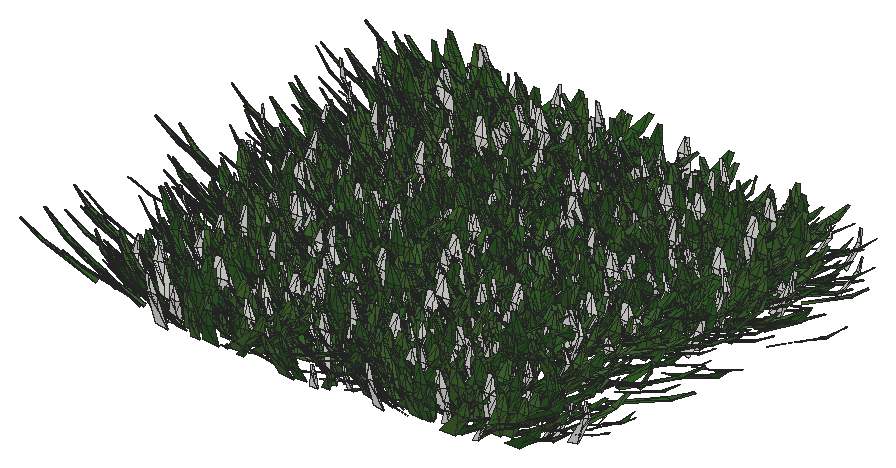
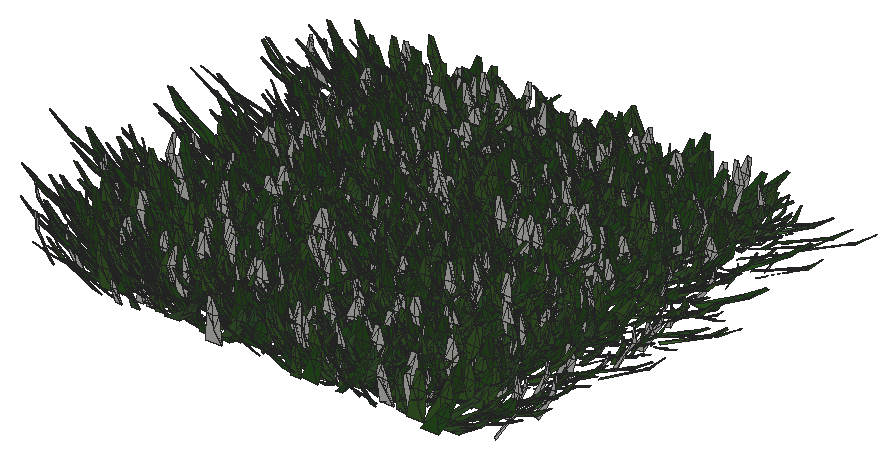
# SketchUp Ruby script. Lengths in inches.
U = 1.inch
M = Sketchup.active_model
def pt(a) = Geom::Point3d.new(a.map { |v| v * U })
def face(e, loops, mat)
  f = e.add_face(loops[0].map { |a| pt(a) })
  loops[1..].each { |l| e.add_face(l.map { |a| pt(a) }).erase! }
  f.material = f.back_material = mat if mat
  f
end
# faces: each face lists its corners as indices into pts; further lists are holes
def faces(e, pts, list, mat = nil) = list.each { |f| face(e, (f[0].is_a?(Array) ? f : [f]).map { |l| l.map { |i| pts[i] } }, mat) }
# xy, xz, yz: faces in a plane at the given z, y or x. An outline is a flat list of corners, or four numbers for a rectangle; further outlines are holes
def ring(l) = l.size == 4 ? [[l[0], l[1]], [l[2], l[1]], [l[2], l[3]], [l[0], l[3]]] : l.each_slice(2).to_a
def flat(e, list, mat, &to3) = list.each { |f| face(e, (f[0].is_a?(Array) ? f : [f]).map { |l| ring(l).map { |u, v| to3.(u, v) } }, mat) }
def xy(e, z, list, mat = nil) = flat(e, list, mat) { |x, y| [x, y, z] }
def xz(e, y, list, mat = nil) = flat(e, list, mat) { |x, z| [x, y, z] }
def yz(e, x, list, mat = nil) = flat(e, list, mat) { |y, z| [x, y, z] }
def lines(e, pts, list) = list.each { |a, b| e.add_line(pt(pts[a]), pt(pts[b])) }
# prism: a flat outline (further loops are holes) pulled along v
def prism(e, loops, v, mat = nil)
  f = face(e, loops, mat); d = Geom::Vector3d.new(v.map { |x| x * U })
  f.pushpull(f.normal.samedirection?(d) ? d.length : -d.length)
end
def box(e, o, s, mat = nil) = prism(e, [[o, [o[0] + s[0], o[1], o[2]], [o[0] + s[0], o[1] + s[1], o[2]], [o[0], o[1] + s[1], o[2]]]], [0, 0, s[2]], mat)
def at(x, y, z, deg = 0) = Geom::Transformation.translation(pt([x, y, z])) * Geom::Transformation.rotation(ORIGIN, Z_AXIS, deg.degrees)
def axes(o, x, y, z) = Geom::Transformation.new([*x, 0, *y, 0, *z, 0, *pt(o).to_a, 1])
def part(name) = M.definitions.add(name)
# library, detail: a bought-in or finely detailed component or shape, given as its bounding box
def library(name, o, s) = part(name).tap { |d| box(d.entities, o, s) }
def detail(e, o, s) = box(e.add_group.entities, o, s)
def put(e, d, t, mat = nil) = e.add_instance(d, t).tap { |i| i.material = mat if mat }
def group(e, t, mat = nil) = e.add_group.tap { |g| g.transformation = t; g.material = mat if mat }.entities
root = M.entities
M.materials.add("Material10").color = [48, 100, 38]
M.materials.add("Material3").color = [68, 110, 58]
M.materials.add("Material4").color = [48, 90, 38]
M.materials.add("Material5").color = [68, 110, 48]
M.materials.add("Material6").color = [48, 90, 48]
M.materials.add("Material7").color = [58, 110, 58]
M.materials.add("Material8").color = [58, 90, 38]
M.materials.add("Material9").color = [68, 100, 58]
c1 = part("grass00")
p = [[-0.6875,0.15,0],[-0.56,0.08,5.52],[-0.04,0.03,2.76],[0.48,-0.02,0],[0.35,-0.02,5.52],[-0.1,-0.14,5.52],
  [-0.12,0.65,8.37],[-0.42,0.65,8.37]]
faces(c1.entities,p,[[0,1,2,3],[3,2,4],[1,5,2],[5,4,2],[1,6,5],[4,5,6],[7,6,1]])
c2 = part("Group16\#1")
put(c2.entities,c1,axes([1.44,-0.61,-0.01],[0.05352,0.12609,0],[-0.10704,0.04543,0.07239],[0.06664,-0.02828,0.11628]),"Material6")
put(c2.entities,c1,axes([0.76,-0.15,-0.01],[0.04676,0.24062,0],[-0.23162,0.04501,0.06642],[0.0652,-0.01267,0.23595]),"Material3")
put(c2.entities,c1,axes([0.79,0.01,-0.01],[-0.00606,0.34651,0],[-0.34381,-0.00602,0.0432],[0.04319,0.00076,0.34386]))
put(c2.entities,c1,axes([1,0.23,-0.01],[-0.07192,0.31144,0],[-0.28722,-0.06632,0.1236],[0.12043,0.02781,0.29478]),"Material5")
put(c2.entities,c1,axes([1.66,0.77,-0.01],[-0.13828,0.29651,0],[-0.21551,-0.1005,0.22471],[0.20365,0.09498,0.23779]),"Material10")
put(c2.entities,c1,axes([0.6875,0.52,-0.01],[-0.18126,0.24051,0],[-0.22746,-0.17142,0.09788],[0.07817,0.05891,0.28481]),"Material5")
put(c2.entities,c1,axes([0.68,0.78,-0.01],[-0.215,0.18688,0],[-0.12385,-0.14248,0.21334],[0.13995,0.16101,0.18878]),"Material3")
put(c2.entities,c1,axes([0.56,1,-0.01],[-0.13756,0.07624,0],[-0.06159,-0.11112,0.0927],[0.04494,0.08108,0.12705]),"Material5")
put(c2.entities,c1,axes([0.2,0.64,-0.01],[-0.23729,0.07254,0],[-0.05711,-0.18681,0.153],[0.04473,0.14632,0.19535]),"Material10")
put(c2.entities,c1,axes([0.0625,0.72,-0.01],[-0.28874,0.02525,0],[-0.02179,-0.24916,0.14647],[0.01276,0.14591,0.25012]),"Material3")
put(c2.entities,c1,axes([-0.08,0.62,-0.01],[-0.34089,-0.04187,0],[0.03255,-0.26504,0.216],[-0.02633,0.21439,0.26703]),"Material10")
put(c2.entities,c1,axes([-0.34,0.98,-0.01],[-0.14314,-0.0493,0],[0.04397,-0.12769,0.06843],[-0.02228,0.0647,0.13505]),"Material10")
put(c2.entities,c1,axes([-0.87,1.45,-0.01],[-0.23488,-0.14114,0],[0.13761,-0.22901,0.06087],[-0.03135,0.05217,0.26717]))
put(c2.entities,c1,axes([-0.72,0.77,-0.01],[-0.14208,-0.13251,0],[0.07209,-0.0773,0.16301],[-0.11118,0.11922,0.1057]),"Material10")
put(c2.entities,c1,axes([-0.62,0.43,-0.01],[-0.14845,-0.21203,0],[0.18654,-0.13061,0.12304],[-0.10079,0.07057,0.22772]),"Material3")
put(c2.entities,c1,axes([-0.68,0.29,-0.01],[-0.13639,-0.32136,0],[0.31723,-0.13464,0.05579],[-0.05136,0.0218,0.34462]),"Material4")
put(c2.entities,c1,axes([-0.64,0.125,-0.01],[-0.0458,-0.23569,0],[0.22124,-0.043,0.08276],[-0.08124,0.01579,0.22538]),"Material7")
put(c2.entities,c1,axes([-1.6,-0.03,-0.01],[0.00576,-0.32897,0],[0.27526,0.00482,0.18018],[-0.18015,-0.00315,0.2753]),"Material5")
put(c2.entities,c1,axes([-1.36,-0.31,-0.01],[0.05718,-0.24765,0],[0.18172,0.04196,0.17267],[-0.16825,-0.03885,0.1865]),"Material10")
put(c2.entities,c1,axes([-1.54,-0.72,-0.01],[0.06537,-0.14017,0],[0.13555,0.06321,0.03939],[-0.0357,-0.01665,0.14956]))
put(c2.entities,c1,axes([-1.19,-0.9,-0.01],[0.09597,-0.12735,0],[0.11214,0.08451,0.07557],[-0.06035,-0.04548,0.14042]),"Material9")
put(c2.entities,c1,axes([-0.47,-0.54,-0.01],[0.11588,-0.10072,0],[0.0618,0.0711,0.12124],[-0.07953,-0.0915,0.0942]))
put(c2.entities,c1,axes([-0.47,-0.84,-0.01],[0.11927,-0.0661,0],[0.06603,0.11913,0.00646],[-0.00313,-0.00565,0.13621]),"Material5")
put(c2.entities,c1,axes([-0.38,-1.24,-0.01],[0.28037,-0.08571,0],[0.0618,0.20215,0.20315],[-0.05939,-0.19428,0.21139]),"Material9")
put(c2.entities,c1,axes([-0.06,-0.66,-0.01],[0.22719,-0.01987,0],[0.01247,0.14255,0.17758],[-0.01547,-0.17691,0.1431]),"Material8")
put(c2.entities,c1,axes([0.11,-0.89,-0.01],[0.14882,0.01828,0],[-0.01058,0.08611,0.12229],[0.01491,-0.12138,0.08676]),"Material6")
put(c2.entities,c1,axes([0.25,-0.72,-0.01],[0.20481,0.07053,0],[-0.06206,0.18022,0.10291],[0.03351,-0.0973,0.1906]),"Material6")
put(c2.entities,c1,axes([0.85,-1.42,-0.01],[0.16481,0.09904,0],[-0.09472,0.15762,0.05616],[0.02893,-0.04814,0.18389]),"Material5")
put(c2.entities,c1,axes([1.01,-1.09,-0.01],[0.21858,0.20385,0],[-0.17495,0.1876,0.15339],[0.10462,-0.11218,0.25652]),"Material10")
put(c2.entities,c1,axes([1.01,-0.71,-0.01],[0.08733,0.12473,0],[-0.06445,0.04512,0.13037],[0.1068,-0.07477,0.07867]),"Material6")
c3 = part("Group15\#1")
put(c3.entities,c2,at(0,0,0))
c4 = part("3darcstudiotree_grass00\#1")
put(c4.entities,c3,at(0,0,0))
put(root,c4,axes([193.53,26.9,7.6],[-2.68493,-0.72179,0],[2.74212,-0.63751,-0.03633],[0.19715,-0.04583,1.73438]))
put(root,c4,axes([193.63,25.22,7.6],[-1.94469,-0.81082,0],[3.41072,-0.51128,-0.04451],[0.23926,-0.03587,1.55797]))
put(root,c4,axes([194.18,17.8125,7.6],[-4.38536,-0.48819,0],[1.68539,-0.94622,-0.04343],[0.09225,-0.05179,1.35201]))
put(root,c4,axes([193.89,13.31,7.6],[-0.93763,-1.01509,0],[3.58265,-0.20683,-0.0292],[0.19066,-0.01101,1.53984]))
put(root,c4,axes([193.6,18.74,7.6],[2.32628,-1.10135,0],[3.26689,0.43127,-0.03491],[0.22091,0.02916,1.65255]))
put(root,c4,axes([194.4,5.27,7.6],[-3.78007,0.18751,0],[-0.9942,-1.25267,-0.05548],[-0.05563,-0.0701,1.6451]))
put(root,c4,axes([195.64,33.04,7.6],[-3.41877,-0.81095,0],[3.11222,-0.82002,-0.00166],[0.00704,-0.00186,1.74215]))
put(root,c4,axes([193.625,37.75,7.6],[3.56011,0.3766,0],[-1.5529,0.91751,-0.02719],[-0.08207,0.04849,1.929]))
put(root,c4,axes([193.64,38.23,7.6],[-0.28146,1.0454,0],[-4.85505,-0.0817,-0.01753],[-0.10805,-0.00182,1.87889]))
put(root,c4,axes([193.54,23.21,7.6],[4.34869,0.47354,0],[-1.70545,0.97885,-0.04191],[-0.08317,0.04774,1.32656]))
put(root,c4,axes([194.17,42.1875,7.6],[0.50605,0.98572,0],[-4.41784,0.14175,-0.0516],[-0.36721,0.01178,1.99718]))
put(root,c4,axes([193.98,29.9,7.6],[4.51798,0.20316,0],[-0.79252,1.10155,-0.03729],[-0.03789,0.05267,1.60628]))
put(root,c4,axes([195.89,11.21,7.6],[-4.34417,-0.18262,0],[0.70687,-1.05094,-0.0114],[0.01401,-0.02082,1.97478]))
put(root,c4,axes([194.25,27.89,7.6],[2.21014,1.15532,0],[-3.78234,0.45223,-0.02212],[-0.14871,0.01778,1.95299]))
put(root,c4,axes([194.5625,16.51,7.6],[-0.29005,1.03921,0],[-4.26068,-0.07432,-0.02357],[-0.13601,-0.00237,1.54387]))
put(root,c4,axes([194.57,9.76,7.6],[4.64548,-0.02052,0],[0.0884,1.25077,-0.02875],[0.00253,0.03584,1.55972]))
put(root,c4,axes([194.73,34.38,7.6],[2.69774,0.60172,0],[-2.53829,0.71125,-0.00625],[-0.03018,0.00846,1.72796]))
put(root,c4,axes([196.32,21.58,7.6],[-4.15604,0.63305,0],[-2.33124,-0.95655,-0.05764],[-0.19304,-0.07921,1.8024]))
put(root,c4,axes([196.75,6.94,7.6],[1.24811,-0.98204,0],[4.93225,0.39179,-0.03698],[0.19941,0.01584,1.82987]))
put(root,c4,axes([197.36,14.11,7.6],[-2.73285,-0.87798,0],[3.13409,-0.60971,-0.01663],[0.09994,-0.01944,1.89037]))
put(root,c4,axes([196.96,4.1,7.6],[-3.26487,0.7652,0],[-2.88539,-0.76944,-0.04557],[-0.23173,-0.0618,1.96028]))
put(root,c4,axes([196.54,30.82,7.6],[-2.34155,0.84913,0],[-3.4682,-0.59774,-0.02321],[-0.12342,-0.02127,1.70026]))
put(root,c4,axes([197.26,8.99,7.6],[-3.68799,0.26675,0],[-1.34322,-1.16069,-0.00573],[-0.00843,-0.00729,1.59925]))
put(root,c4,axes([197.2,36.07,7.6],[2.33049,-0.73294,0],[3.96124,0.7872,-0.06111],[0.26943,0.05354,1.78135]))
put(root,c4,axes([197.32,40.72,7.6],[3.80611,-0.44418,0],[1.98468,1.06289,-0.02938],[0.0699,0.03743,1.64954]))
put(root,c4,axes([197.125,20.72,7.6],[5.11514,-0.08131,0],[0.26106,1.02638,-0.03177],[0.01497,0.05885,1.90853]))
put(root,c4,axes([199.55,25.45,7.6],[-4.00581,-0.59681,0],[2.18474,-0.9165,-0.01663],[0.06212,-0.02606,1.94585]))
put(root,c4,axes([199.72,4.14,7.6],[3.537,-0.94689,0],[2.76209,0.64485,-0.01281],[0.06208,0.01449,1.56626]))
put(root,c4,axes([201.32,22.05,7.6],[-1.77,-0.83286,0],[4.02387,-0.53447,-0.00698],[0.04087,-0.00543,1.8873]))
put(root,c4,axes([200.93,6.76,7.6],[1.67638,-1.0425,0],[4.59893,0.4622,-0.01772],[0.09487,0.00953,1.7874]))
put(root,c4,axes([201.5,13.21,7.6],[-3.4263,-0.91381,0],[3.1573,-0.73989,-0.03051],[0.13581,-0.03183,1.65027]))
put(root,c4,axes([200.84,39.84,7.6],[2.30637,-1.06411,0],[3.89478,0.5276,-0.00988],[0.05923,0.00802,1.88737]))
put(root,c4,axes([199.71,17.35,7.6],[5.17876,0.00972,0],[-0.03633,1.20929,-0.012],[-0.00051,0.01694,1.70791]))
put(root,c4,axes([200.52,5.41,7.6],[3.44483,-0.53348,0],[2.02838,0.81862,-0.00486],[0.01517,0.00612,1.42853]))
put(root,c4,axes([199.85,19.01,7.6],[1.61317,1.05687,0],[-3.89248,0.37133,-0.03212],[-0.19954,0.01904,1.73128]))
put(root,c4,axes([200.26,9.9,7.6],[4.23132,0.05428,0],[-0.26252,1.27912,-0.05168],[-0.01396,0.06804,1.68853]))
put(root,c4,axes([200.07,14.6,7.6],[0.18775,1.28338,0],[-5.04354,0.04611,-0.0182],[-0.08343,0.00076,1.44668]))
put(root,c4,axes([200.24,27.72,7.6],[0.66659,0.99759,0],[-3.70369,0.15468,-0.00028],[-0.00179,0.00007,1.50491]))
put(root,c4,axes([200.59,38.79,7.6],[-0.12653,1.00906,0],[-4.40907,-0.03456,-0.04067],[-0.22619,-0.00177,1.53414]))
put(root,c4,axes([201.48,32.94,7.6],[-3.44749,0.85218,0],[-2.82175,-0.71346,-0.03762],[-0.15511,-0.03922,1.47105]))
put(root,c4,axes([200.23,36.24,7.6],[0.53467,1.10303,0],[-5.00046,0.15149,-0.01569],[-0.0735,0.00223,1.48562]))
put(root,c4,axes([202.59,29.92,7.6],[-3.66347,-0.90665,0],[3.59625,-0.9082,-0.03717],[0.1584,-0.04,1.93537]))
put(root,c4,axes([202.37,26.35,7.6],[-4.4143,-0.18542,0],[0.67487,-1.00419,-0.01654],[0.02043,-0.03039,1.89711]))
put(root,c4,axes([202.8,30.91,7.6],[-1.79213,-0.89815,0],[3.71156,-0.46287,-0.00448],[0.02956,-0.00369,1.90991]))
put(root,c4,axes([201.9,16.58,7.6],[-3.49749,0.50247,0],[-2.5408,-1.10534,-0.04948],[-0.12396,-0.05393,1.60238]))
put(root,c4,axes([201.3,34.43,7.6],[0.73607,0.9032,0],[-4.03456,0.2055,-0.04728],[-0.29589,0.01507,1.64346]))
put(root,c4,axes([201.66,23.49,7.6],[3.54729,0.43846,0],[-1.7678,0.89387,-0.03066],[-0.09543,0.04825,1.75054]))
put(root,c4,axes([202.87,8.96,7.6],[0.42302,-0.9917,0],[3.83549,0.10225,-0.04937],[0.35058,0.00935,1.72169]))
put(root,c4,axes([203.12,20.35,7.6],[-1.77196,1.05602,0],[-3.98674,-0.4181,-0.04701],[-0.29505,-0.03094,1.83905]))
put(root,c4,axes([203.33,11.55,7.6],[0.45093,1.12107,0],[-3.84241,0.0966,-0.04963],[-0.30261,0.00761,1.47912]))
put(root,c4,axes([202.64,41.44,7.6],[3.32772,0.78374,0],[-3.41591,0.90649,-0.01047],[-0.04436,0.01177,1.92288]))
put(root,c4,axes([203.77,36.9,7.6],[4.23567,0.36269,0],[-1.24548,0.90909,-0.02009],[-0.04731,0.03453,1.7458]))
put(root,c4,axes([205.65,36.125,7.6],[-4.4227,-0.30365,0],[1.03811,-0.94502,-0.02848],[0.05651,-0.05144,1.83531]))
put(root,c4,axes([205.36,40.33,7.6],[-0.43672,-1.24202,0],[4.36716,-0.09597,-0.04765],[0.30496,-0.0067,1.76037]))
put(root,c4,axes([205.6,42.0625,7.6],[-4.11211,0.64037,0],[-1.92557,-0.77282,-0.01072],[-0.04599,-0.01846,1.84718]))
put(root,c4,axes([206.2,14.46,7.6],[-4.34593,0.58001,0],[-2.21528,-1.03742,-0.03463],[-0.1032,-0.04833,1.86049]))
put(root,c4,axes([205.74,19.26,7.6],[-1.86227,1.06204,0],[-3.42788,-0.37567,-0.01229],[-0.09526,-0.01044,1.9803]))
put(root,c4,axes([207.29,34.14,7.6],[-3.5926,-0.75101,0],[3.19063,-0.95393,-0.04137],[0.11689,-0.03495,1.36909]))
put(root,c4,axes([206.76,28.27,7.6],[3.48166,-0.50059,0],[2.44605,1.06327,-0.03788],[0.08627,0.0375,1.40078]))
put(root,c4,axes([206.13,26.41,7.6],[4.43547,0.23328,0],[-0.86743,1.0308,-0.04482],[-0.053,0.06298,1.51278]))
put(root,c4,axes([208.07,37.01,7.6],[-3.11664,-0.68281,0],[2.49826,-0.71269,-0.01406],[0.06937,-0.01979,1.77353]))
put(root,c4,axes([207.15,32.86,7.6],[4.18182,-0.37358,0],[1.54336,1.07977,-0.0155],[0.03636,0.02544,1.9985]))
put(root,c4,axes([208.6,10.53,7.6],[-2.65841,-0.80925,0],[2.97739,-0.6113,-0.021],[0.09455,-0.01941,1.40308]))
put(root,c4,axes([208.53,15.63,7.6],[-1.89766,-0.97867,0],[3.50817,-0.42515,-0.03263],[0.22536,-0.02731,1.87]))
put(root,c4,axes([207.34,31.4,7.6],[3.92204,-0.31031,0],[1.16336,0.91899,-0.04021],[0.0777,0.06138,1.5432]))
put(root,c4,axes([208.71,13.54,7.6],[-4.71443,0.13943,0],[-0.55237,-1.16732,-0.02284],[-0.01323,-0.02795,1.44864]))
put(root,c4,axes([208.12,8.21,7.6],[-2.39721,0.74853,0],[-3.19848,-0.64021,-0.02462],[-0.14683,-0.02939,1.95656]))
put(root,c4,axes([207.49,5.93,7.6],[3.23025,0.97107,0],[-3.57979,0.74426,-0.02991],[-0.15449,0.03212,1.95467]))
put(root,c4,axes([209.52,20.78,7.6],[0.02853,-0.96411,0],[5.08808,0.00941,-0.04606],[0.26224,0.00049,1.81052]))
put(root,c4,axes([207.8,21.97,7.6],[3.66614,0.51192,0],[-1.98914,0.89033,-0.02091],[-0.0622,0.02784,1.55496]))
put(root,c4,axes([207.7,29.71,7.6],[4.6069,0.58631,0],[-2.28752,1.12337,-0.01612],[-0.03759,0.01846,1.61949]))
put(root,c4,axes([209.28,24.07,7.6],[-3.88433,0.51238,0],[-1.98517,-0.9406,-0.01893],[-0.04557,-0.02159,1.37131]))
put(root,c4,axes([209.31,7.3,7.6],[-3.68297,0.59369,0],[-2.11941,-0.82173,-0.01497],[-0.04852,-0.01881,1.4615]))
put(root,c4,axes([208.62,3.97,7.6],[0.49612,1.17734,0],[-3.69255,0.09725,-0.01763],[-0.12152,0.0032,1.60818]))
put(root,c4,axes([208.87,25,7.6],[3.11929,0.72453,0],[-2.48773,0.6694,-0.03885],[-0.22621,0.06087,1.95422]))
put(root,c4,axes([209.44,38.55,7.6],[3.97995,-0.28298,0],[1.30466,1.14685,-0.03545],[0.05768,0.0507,1.77295]))
put(root,c4,axes([209.12,17.48,7.6],[0.95512,1.24392,0],[-4.78219,0.22949,-0.02457],[-0.12659,0.00607,1.59681]))
put(root,c4,axes([209.75,11.13,7.6],[4.18474,0.7675,0],[-2.60572,0.88797,-0.00415],[-0.01182,0.00403,1.32509]))
put(root,c4,axes([211.4375,14.88,7.6],[1.49904,-0.99382,0],[4.36571,0.41157,-0.04892],[0.30393,0.02865,1.93615]))
put(root,c4,axes([212.16,28.19,7.6],[-3.34703,-0.44034,0],[1.86344,-0.88525,-0.01604],[0.05682,-0.02699,1.9024]))
put(root,c4,axes([212.32,34.26,7.6],[-0.87549,-1.06671,0],[4.68602,-0.24038,-0.03341],[0.20374,-0.01045,1.86102]))
put(root,c4,axes([211.93,13.05,7.6],[1.68499,-1.00901,0],[4.65536,0.48589,-0.03949],[0.20736,0.02164,1.7941]))
put(root,c4,axes([212.65,22.62,7.6],[-2.77219,-0.80321,0],[3.53234,-0.76197,-0.03179],[0.10998,-0.02372,1.33245]))
put(root,c4,axes([213.21,30.65,7.6],[0.45917,-1.01545,0],[5.11405,0.14453,-0.01256],[0.07404,0.00209,1.90836]))
put(root,c4,axes([211.53,7.4,7.6],[3.91432,0.2962,0],[-1.14145,0.94277,-0.0422],[-0.0933,0.07706,1.87907]))
put(root,c4,axes([211.99,23.08,7.6],[4.97696,-0.05302,0],[0.19507,1.14438,-0.04096],[0.01048,0.0615,1.72127]))
put(root,c4,axes([213.94,17.72,7.6],[-1.27908,-0.88935,0],[3.91716,-0.35211,-0.0171],[0.11094,-0.00997,1.79343]))
put(root,c4,axes([213.54,40.375,7.6],[-4.79032,0.48606,0],[-1.70961,-1.05304,-0.01879],[-0.03655,-0.02252,1.46955]))
put(root,c4,axes([213.89,11.72,7.6],[-3.54874,-0.19762,0],[0.84752,-0.95118,-0.02543],[0.03659,-0.04107,1.61262]))
put(root,c4,axes([213.27,32.93,7.6],[-3.16014,0.66861,0],[-3.08586,-0.91157,-0.05904],[-0.18903,-0.05584,1.47981]))
put(root,c4,axes([214.12,9.9,7.6],[1.28054,-1.03018,0],[4.2523,0.33036,-0.02169],[0.11477,0.00892,1.54236]))
put(root,c4,axes([214.62,7.89,7.6],[-0.71824,-1.02023,0],[5.03908,-0.22172,-0.05842],[0.35675,-0.0157,1.98292]))
put(root,c4,axes([213.74,25.68,7.6],[4.32394,-0.4782,0],[1.59071,0.89896,-0.00969],[0.0217,0.01226,1.36001]))
put(root,c4,axes([215.21,20.29,7.6],[-4.09477,-0.54974,0],[1.8737,-0.87227,-0.0264],[0.09985,-0.04648,1.979]))
put(root,c4,axes([215.04,38.31,7.6],[-4.29836,-0.05077,0],[0.23538,-1.24557,-0.03065],[0.00914,-0.04835,1.9691]))
put(root,c4,axes([213.28,27.02,7.6],[4.80121,0.29914,0],[-1.24856,1.25248,-0.03274],[-0.0398,0.03992,1.62193]))
put(root,c4,axes([215.37,16.01,7.6],[-3.91367,-0.4767,0],[2.06304,-1.05859,-0.02869],[0.08103,-0.04158,1.89824]))
put(root,c4,axes([213.72,18.55,7.6],[4.81743,-0.02087,0],[0.06672,0.96257,-0.04649],[0.00527,0.07597,1.57333]))
put(root,c4,axes([214.55,41.58,7.6],[4.37292,-0.40538,0],[1.54259,1.04001,-0.01564],[0.037,0.02495,1.88746]))
put(root,c4,axes([214.67,36.68,7.6],[-1.42316,0.86255,0],[-3.977,-0.41012,-0.01866],[-0.09986,-0.0103,1.55626]))
put(root,c4,axes([215.33,29.46,7.6],[5.06053,-0.0101,0],[0.03814,1.19402,-0.00522],[0.0002,0.00625,1.42947]))
put(root,c4,axes([215.54,35.44,7.6],[1.90816,0.82105,0],[-3.58285,0.52042,-0.03711],[-0.20984,0.03048,1.69359]))
put(root,c4,axes([215.37,5.03,7.6],[2.85091,0.72979,0],[-2.82823,0.69053,-0.01838],[-0.08823,0.02154,1.65818]))
put(root,c4,axes([217.7,19.23,7.6],[-4.57395,-0.56919,0],[2.24978,-1.12995,-0.0574],[0.11462,-0.05757,1.41402]))
put(root,c4,axes([218.06,40.03,7.6],[-4.36386,0.0424,0],[-0.14663,-0.94321,-0.04521],[-0.01421,-0.09143,1.91035]))
put(root,c4,axes([218.53,32.79,7.6],[-3.84808,-0.62814,0],[2.34387,-0.89743,-0.0556],[0.18939,-0.07251,1.66946]))
put(root,c4,axes([217.5,23.94,7.6],[-2.81015,0.82442,0],[-3.69627,-0.78745,-0.01912],[-0.06485,-0.01382,1.35238]))
put(root,c4,axes([218.8,11.21,7.6],[-3.5015,-0.36139,0],[1.44415,-0.87453,-0.01181],[0.03303,-0.02,1.73426]))
put(root,c4,axes([218.63,17.63,7.6],[-0.56459,-1.01387,0],[4.32656,-0.15058,-0.04493],[0.31224,-0.01087,1.91565]))
put(root,c4,axes([218.73,38.4375,7.6],[0.89168,-0.93114,0],[3.99265,0.23897,-0.00366],[0.02101,0.00126,1.51551]))
put(root,c4,axes([219.31,10.53,7.6],[0.23484,-1.14494,0],[3.96232,0.0508,-0.01161],[0.06761,0.00087,1.44612]))
put(root,c4,axes([219.99,28.65,7.6],[-3.5181,-0.78299,0],[2.9623,-0.83188,-0.03256],[0.12635,-0.03548,1.62483]))
put(root,c4,axes([220.08,31.54,7.6],[-3.94189,0.10624,0],[-0.456,-1.0575,-0.01956],[-0.01557,-0.0361,1.97453]))
put(root,c4,axes([218.7,5.51,7.6],[-0.1159,1.07064,0],[-4.16097,-0.02815,-0.00627],[-0.03911,-0.00026,1.62459]))
put(root,c4,axes([220.65,41.44,7.6],[-2.63935,-0.88257,0],[3.19573,-0.59731,-0.02089],[0.10644,-0.01989,1.58683]))
put(root,c4,axes([219.96,14.6,7.6],[-3.39832,0.86181,0],[-2.85508,-0.70364,-0.05097],[-0.26206,-0.06459,1.80901]))
put(root,c4,axes([219.55,4.17,7.6],[-2.0463,0.79301,0],[-3.44855,-0.55617,-0.00439],[-0.02397,-0.00387,1.66469]))
put(root,c4,axes([219.52,37.24,7.6],[-1.30702,1.14892,0],[-3.96735,-0.28208,-0.01558],[-0.11053,-0.00786,1.90128]))
put(root,c4,axes([219.08,21.61,7.6],[3.62958,0.6733,0],[-2.52662,0.85126,-0.02502],[-0.10717,0.03611,1.90511]))
put(root,c4,axes([221.32,35.69,7.6],[-1.1386,-0.97265,0],[4.79603,-0.3509,-0.04795],[0.2257,-0.01651,1.53186]))
put(root,c4,axes([219.74,8.16,7.6],[-0.88584,1.09832,0],[-4.93295,-0.24867,-0.03197],[-0.17795,-0.00897,1.78572]))
put(root,c4,axes([221.17,6.98,7.6],[-3.95588,0.56377,0],[-2.45949,-1.07862,-0.01918],[-0.05514,-0.02418,1.80194]))
put(root,c4,axes([221.22,20.24,7.6],[1.93293,-0.87029,0],[3.69238,0.51255,-0.03203],[0.18787,0.02608,1.771]))
put(root,c4,axes([221.1,34.72,7.6],[-3.12402,0.89295,0],[-3.68078,-0.80483,-0.03347],[-0.1578,-0.0345,1.91416]))
put(root,c4,axes([220.48,15.49,7.6],[4.8764,0.03202,0],[-0.108,1.02786,-0.04419],[-0.00896,0.08526,1.98467]))
put(root,c4,axes([221.96,29.5625,7.6],[-4.39634,0.48093,0],[-1.83375,-1.04768,-0.02625],[-0.05381,-0.03075,1.46233]))
put(root,c4,axes([221.1,24.78,7.6],[-0.42678,0.97311,0],[-4.0579,-0.11123,-0.02456],[-0.16336,-0.00448,1.70727]))
put(root,c4,axes([221.05,12.89,7.6],[5.0854,0.12715,0],[-0.47106,1.17748,-0.02551],[-0.01271,0.03178,1.48132]))
put(root,c4,axes([221.6875,26.26,7.6],[3.65373,-0.31511,0],[1.20707,0.87477,-0.03311],[0.07347,0.05325,1.57439]))
put(root,c4,axes([224.05,34.74,7.6],[-4.47721,-0.33604,0],[1.36403,-1.13585,-0.01736],[0.02251,-0.01875,1.33702]))
put(root,c4,axes([223.86,21.88,7.6],[1.8365,-1.07849,0],[4.69569,0.49975,-0.03539],[0.15489,0.01648,1.51703]))
put(root,c4,axes([224.35,32.42,7.6],[-2.97525,-0.81655,0],[2.97657,-0.67786,-0.02128],[0.12207,-0.0278,1.95268]))
put(root,c4,axes([224.625,7.9,7.6],[-3.29866,-0.81098,0],[2.55083,-0.64847,-0.00764],[0.04274,-0.01087,1.81511]))
put(root,c4,axes([224.67,40.375,7.6],[0.28036,-1.11473,0],[4.12363,0.06482,-0.00515],[0.03488,0.00055,1.75106]))
put(root,c4,axes([223.58,25.47,7.6],[-2.06266,0.86143,0],[-3.87268,-0.57956,-0.03562],[-0.14938,-0.02236,1.37892]))
put(root,c4,axes([224.375,5.95,7.6],[0.38604,-0.97045,0],[3.84574,0.09561,-0.03727],[0.26595,0.00661,1.73202]))
put(root,c4,axes([224.67,9.9375,7.6],[-3.76521,0.1423,0],[-0.75972,-1.25635,-0.03474],[-0.02334,-0.0386,1.42794]))
put(root,c4,axes([223.64,16.19,7.6],[-0.0845,1.11929,0],[-4.4686,-0.02108,-0.05443],[-0.30573,-0.00144,1.56933]))
put(root,c4,axes([225.33,31.15,7.6],[1.4049,-0.85059,0],[4.43609,0.45793,-0.04448],[0.26457,0.02731,1.93016]))
put(root,c4,axes([225.625,36.97,7.6],[-0.32645,-1.07416,0],[4.58767,-0.08714,-0.05563],[0.36288,-0.00689,1.88098]))
put(root,c4,axes([225.45,29.23,7.6],[-0.59232,1.12492,0],[-3.6265,-0.11934,-0.03263],[-0.21174,-0.00697,1.49628]))
put(root,c4,axes([225.66,28.16,7.6],[4.0581,-0.29722,0],[1.26127,1.0763,-0.01036],[0.0201,0.01715,1.93559]))
